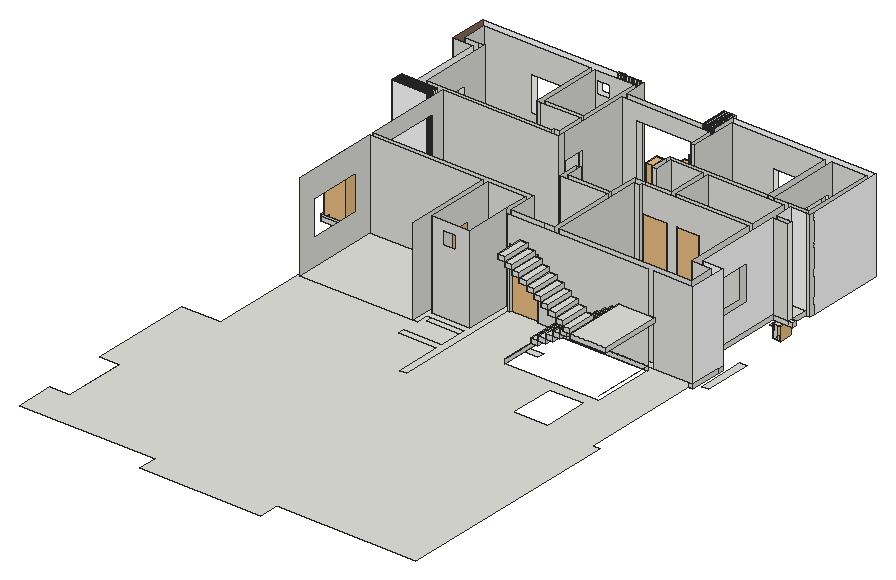
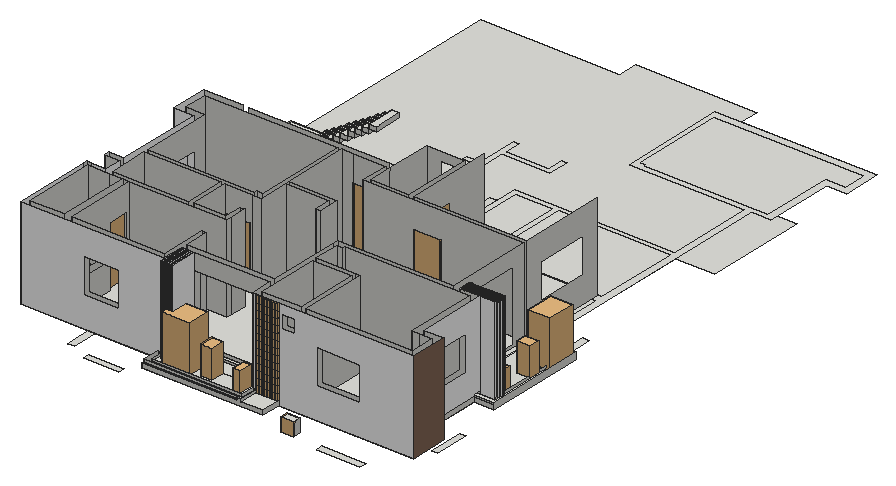
# SketchUp Ruby script. Lengths in inches.
U = 1.inch
M = Sketchup.active_model
def pt(a) = Geom::Point3d.new(a.map { |v| v * U })
def face(e, loops, mat)
  f = e.add_face(loops[0].map { |a| pt(a) })
  loops[1..].each { |l| e.add_face(l.map { |a| pt(a) }).erase! }
  f.material = f.back_material = mat if mat
  f
end
# faces: each face lists its corners as indices into pts; further lists are holes
def faces(e, pts, list, mat = nil) = list.each { |f| face(e, (f[0].is_a?(Array) ? f : [f]).map { |l| l.map { |i| pts[i] } }, mat) }
# xy, xz, yz: faces in a plane at the given z, y or x. An outline is a flat list of corners, or four numbers for a rectangle; further outlines are holes
def ring(l) = l.size == 4 ? [[l[0], l[1]], [l[2], l[1]], [l[2], l[3]], [l[0], l[3]]] : l.each_slice(2).to_a
def flat(e, list, mat, &to3) = list.each { |f| face(e, (f[0].is_a?(Array) ? f : [f]).map { |l| ring(l).map { |u, v| to3.(u, v) } }, mat) }
def xy(e, z, list, mat = nil) = flat(e, list, mat) { |x, y| [x, y, z] }
def xz(e, y, list, mat = nil) = flat(e, list, mat) { |x, z| [x, y, z] }
def yz(e, x, list, mat = nil) = flat(e, list, mat) { |y, z| [x, y, z] }
def lines(e, pts, list) = list.each { |a, b| e.add_line(pt(pts[a]), pt(pts[b])) }
# prism: a flat outline (further loops are holes) pulled along v
def prism(e, loops, v, mat = nil)
  f = face(e, loops, mat); d = Geom::Vector3d.new(v.map { |x| x * U })
  f.pushpull(f.normal.samedirection?(d) ? d.length : -d.length)
end
def box(e, o, s, mat = nil) = prism(e, [[o, [o[0] + s[0], o[1], o[2]], [o[0] + s[0], o[1] + s[1], o[2]], [o[0], o[1] + s[1], o[2]]]], [0, 0, s[2]], mat)
def at(x, y, z, deg = 0) = Geom::Transformation.translation(pt([x, y, z])) * Geom::Transformation.rotation(ORIGIN, Z_AXIS, deg.degrees)
def axes(o, x, y, z) = Geom::Transformation.new([*x, 0, *y, 0, *z, 0, *pt(o).to_a, 1])
def part(name) = M.definitions.add(name)
# library, detail: a bought-in or finely detailed component or shape, given as its bounding box
def library(name, o, s) = part(name).tap { |d| box(d.entities, o, s) }
def detail(e, o, s) = box(e.add_group.entities, o, s)
def put(e, d, t, mat = nil) = e.add_instance(d, t).tap { |i| i.material = mat if mat }
def group(e, t, mat = nil) = e.add_group.tap { |g| g.transformation = t; g.material = mat if mat }.entities
root = M.entities
M.materials.add("Manhattan Creative Coating ML 1016B 24.75cm").color = [255, 255, 255]
M.materials.add("Wintan - wpa36452 29.79cm").color = [255, 255, 255]
M.materials.add("Wood Planks C01 100cm\#1").color = [136, 107, 89]
c1 = part("Stair tread \#1")
box(c1.entities,[0,0,0],[10,39,7])
c2 = part("Stair tread")
box(c2.entities,[0,0,0],[10,39,7])
c3 = part("Group\#13")
box(c3.entities,[100,0,63],[49,84,7])
put(c3.entities,c1,at(50,45,28))
put(c3.entities,c1,at(20,45,7))
put(c3.entities,c1,at(90,45,56))
put(c3.entities,c1,at(70,45,42))
put(c3.entities,c1,at(40,45,21))
put(c3.entities,c1,at(60,45,35))
put(c3.entities,c1,at(10,45,0))
put(c3.entities,c1,at(30,45,14))
put(c3.entities,c1,at(80,45,49))
put(c3.entities,c2,at(90,0,70))
put(c3.entities,c2,at(10,0,126))
put(c3.entities,c2,at(60,0,91))
put(c3.entities,c2,at(30,0,112))
put(c3.entities,c2,at(50,0,98))
put(c3.entities,c2,at(70,0,84))
put(c3.entities,c2,at(80,0,77))
put(c3.entities,c2,at(40,0,105))
put(c3.entities,c2,at(0,0,133))
put(c3.entities,c2,at(20,0,119))
c4 = library("Door 243 053",[-21.6,-2.79,-0.07],[43.2,5.58,82.64])
c5 = library("Potted Plant 02",[-16.98,-19.78,0],[30.04,38.68,37.52])
c6 = library("Tlon Light 650 Ceiling 152 007",[-12.8,-12.8,-3.78],[25.6,25.6,3.58])
c7 = part("Square rail bar")
box(c7.entities,[0,0,-1],[51.7,1,1])
c8 = part("Group\#20")
xy(c8.entities,0,[[0,0,51.7,106.6]])
xy(c8.entities,1,[[0,0,51.7,107.6]])
xz(c8.entities,0,[[0,0,51.7,1]])
xz(c8.entities,107.6,[[0,0,51.7,1]])
yz(c8.entities,0,[[0,0,107.6,1]])
yz(c8.entities,51.7,[[0,0,107.6,1]])
put(c8.entities,c7,at(0,106.6,0))
put(c8.entities,c7,at(0,0,0))
put(c8.entities,c7,at(0,103.05,0))
put(c8.entities,c7,at(0,99.49,0))
put(c8.entities,c7,at(0,95.94,0))
put(c8.entities,c7,at(0,92.39,0))
put(c8.entities,c7,at(0,88.83,0))
put(c8.entities,c7,at(0,85.28,0))
put(c8.entities,c7,at(0,81.73,0))
put(c8.entities,c7,at(0,78.17,0))
put(c8.entities,c7,at(0,74.62,0))
put(c8.entities,c7,at(0,71.07,0))
put(c8.entities,c7,at(0,67.51,0))
put(c8.entities,c7,at(0,63.96,0))
put(c8.entities,c7,at(0,60.41,0))
put(c8.entities,c7,at(0,56.85,0))
put(c8.entities,c7,at(0,53.3,0))
put(c8.entities,c7,at(0,49.75,0))
put(c8.entities,c7,at(0,46.19,0))
put(c8.entities,c7,at(0,42.64,0))
put(c8.entities,c7,at(0,39.09,0))
put(c8.entities,c7,at(0,35.53,0))
put(c8.entities,c7,at(0,31.98,0))
put(c8.entities,c7,at(0,28.43,0))
put(c8.entities,c7,at(0,24.875,0))
put(c8.entities,c7,at(0,21.32,0))
put(c8.entities,c7,at(0,17.77,0))
put(c8.entities,c7,at(0,14.21,0))
put(c8.entities,c7,at(0,10.66,0))
put(c8.entities,c7,at(0,7.11,0))
put(c8.entities,c7,at(0,3.55,0))
put(c8.entities,c7,at(0,0,0))
c9 = library("Potted Plant 13",[-10,-7.28,0],[18.93,15.17,39.22])
c10 = library("Potted Plant 50-12",[-6.11,-5.26,0],[11.24,10.56,13.41])
c11 = part("Rectangular column")
box(c11.entities,[0,16,0],[27,1,119.8])
box(c11.entities,[0,3.56,0],[27,1,120])
box(c11.entities,[0,1.78,0],[27,1,120])
box(c11.entities,[0,14.22,0],[27,1,119.8])
box(c11.entities,[0,5.33,0],[27,1,120])
box(c11.entities,[0,7.11,0],[27,1,120])
box(c11.entities,[0,10.67,0],[27,1,120.2])
box(c11.entities,[0,12.44,0],[27,1,119.8])
box(c11.entities,[0,0,0],[27,1,120])
xy(c11.entities,0,[[0,8.89,27,9.89]])
xy(c11.entities,120,[[0,8.89,27,9.89]])
xz(c11.entities,8.89,[[0,0,27,120]])
xz(c11.entities,9.89,[[0,0,27,120]])
yz(c11.entities,0,[[8.89,0,9.89,120]],"Wintan - wpa36452 29.79cm")
yz(c11.entities,27,[[8.89,0,9.89,120]])
c12 = library("Window Crafter Awning 2",[0,-9.5,0],[17.5,11.27,18])
c13 = part("Decorative grille insert")
p = [[0.961,0,5],[0.961,0,4.995]]
lines(c13.entities,p,[[0,1]])
detail(c13.entities,[0,0,0],[4.12,1.8,10])
xy(root,336,[[1843.02,926.67,1852.02,998.67],[2008.02,962.67,2014.02,986.67],[2078.52,980.67,2117.52,989.67],[1966.02,1022.67,2002.02,1028.67],[2294.52,1040.67,2303.52,1106.67],
  [2149.02,1121.67,2181.02,1127.67],[2195.52,1121.67,2225.52,1127.67],[2005.02,1160.17,2011.02,1190.17],[1816.02,1172.67,1825.02,1220.67],[2267.52,1190.67,2276.52,1220.67],
  [1954.02,1193.67,1978.02,1199.67],[2267.52,1232.67,2276.52,1280.67],[1863.02,1286.67,1923.02,1295.67],[2195.52,1286.67,2243.52,1295.67]])
xy(root,342,[[2029.77,917.67,2047.27,926.67],[2294.52,1162.17,2303.52,1179.67],[1953.02,1286.67,1970.52,1295.67]])
xy(root,351,[[1843.02,1046.67,1852.02,1130.67],[2031.27,1256.67,2115.27,1265.67]])
xy(root,360,[[2294.52,1162.17,2303.52,1179.67],[1953.02,1286.67,1970.52,1295.67]])
xy(root,372,[[[1975.05,473.67,1975.05,500.67,1789.02,500.67,1789.02,551.67,1816.02,551.67,1816.02,637.17,1789.02,637.17,1789.02,778.17,1843.02,778.17,1843.02,1018.17,1789.02,1018.17,1789.02,1159.17,1816.02,1159.17,1816.02,1244.67,1789.02,1244.67,1789.02,1295.67,1975.05,1295.67,1975.05,1322.67,2141.52,1322.67,2141.52,1295.67,2330.52,1295.67,2330.52,1181.67,2324.52,1181.67,2324.52,1157.7,2330.52,1157.7,2330.52,1151.7,2303.52,1151.7,2303.52,1031.67,2330.52,1031.67,2330.52,980.67,2324.52,980.67,2324.52,815.67,2333.52,815.67,2333.52,500.67,2141.52,500.67,2141.52,473.67],[2138.52,896.67,2267.52,980.67],[2211.52,819.67,2259.52,883.67]],[[1789.02,500.67,2011.02,500.67,2011.02,647.67,1852.02,647.67,1852.02,767.67,2072.52,767.67,2072.52,806.67,2132.52,806.67,2132.52,715.17,2066.52,715.17,2066.52,686.67,2072.52,686.67,2072.52,709.17,2132.52,709.17,2132.52,686.67,2138.52,686.67,2138.52,743.67,2158.52,743.67,2158.52,749.67,2138.52,749.67,2138.52,806.67,2324.52,806.67,2324.52,815.67,2276.52,815.67,2276.52,980.67,2330.52,980.67,2330.52,1031.67,2303.52,1031.67,2303.52,1151.7,2324.52,1151.7,2324.52,1157.7,2303.52,1157.7,2303.52,1181.67,2330.52,1181.67,2330.52,1295.67,2132.52,1295.67,2132.52,1223.67,2138.52,1223.67,2138.52,1286.67,2324.52,1286.67,2324.52,1187.67,2132.52,1187.67,2132.52,1181.67,2183.52,1181.67,2183.52,1127.67,2132.52,1127.67,2132.52,989.67,2072.52,989.67,2072.52,1028.67,1852.02,1028.67,1852.02,1148.67,2011.02,1148.67,2011.02,1256.67,2132.52,1256.67,2132.52,1265.67,2011.02,1265.67,2011.02,1295.67,1798.02,1295.67,1798.02,1286.67,1945.02,1286.67,1945.02,1193.67,2005.02,1193.67,2005.02,1157.67,1997.02,1157.67,1997.02,1154.67,1825.02,1154.67,1825.02,1253.67,1816.02,1253.67,1816.02,1148.67,1843.02,1148.67,1843.02,647.67,1816.02,647.67,1816.02,551.67,1789.02,551.67],[1852.02,773.67,1852.02,893.67,2014.02,893.67,2014.02,891.17,2017.02,891.17,2017.02,905.17,2014.02,905.17,2014.02,902.67,1852.02,902.67,1852.02,1022.67,2008.02,1022.67,2008.02,902.67,2014.02,902.67,2014.02,1022.67,2066.52,1022.67,2066.52,773.67,2014.02,773.67,2014.02,893.67,2008.02,893.67,2008.02,773.67],[2075.52,815.67,2267.52,980.67],[1798.02,509.67,1798.02,542.67,1825.02,542.67,1825.02,641.67,1997.02,641.67,1997.02,638.67,2005.02,638.67,2005.02,509.67],[2138.52,989.67,2138.52,1118.67,2146.52,1118.67,2146.52,1121.67,2294.52,1121.67,2294.52,1022.67,2321.52,1022.67,2321.52,989.67],[2189.52,1127.67,2294.52,1181.67],[1951.02,1199.67,2005.02,1286.67]],[2014.02,917.67,2066.52,926.67],[2066.52,1081.17,2132.52,1081.17,2132.52,1087.17,2072.52,1087.17,2072.52,1109.67,2066.52,1109.67],[2132.52,1157.67,2138.52,1181.67],
  [2267.52,1187.67,2276.52,1286.67],[1789.02,1244.67,1816.02,1244.67,1816.02,1253.67,1798.02,1253.67,1798.02,1295.67,1789.02,1295.67]])
xy(root,378,[[2066.52,806.67,2075.52,806.67,2075.52,980.67,2078.52,980.67,2078.52,989.67,2072.52,989.67,2072.52,1028.67,2002.02,1028.67,2002.02,1022.67,2008.02,1022.67,2008.02,986.67,2014.02,986.67,2014.02,1022.67,2066.52,1022.67,2066.52,926.67,2014.02,926.67,2014.02,962.67,2008.02,962.67,2008.02,902.67,2014.02,902.67,2014.02,917.67,2066.52,917.67,2066.52,878.67,2014.02,878.67,2014.02,869.67,2066.52,869.67],[1852.02,902.67,2008.02,902.67,2008.02,962.67,2014.02,962.67,2014.02,986.67,2008.02,986.67,2008.02,1022.67,2002.02,1022.67,2002.02,1028.67,1966.02,1028.67,1966.02,1022.67,1852.02,1022.67],[2014.02,926.67,2066.52,1022.67],[2132.52,980.67,2330.52,980.67,2330.52,1022.67,2321.52,1022.67,2321.52,989.67,2138.52,989.67,2138.52,1118.67,2132.52,1118.67],[2072.52,989.67,2132.52,989.67,2132.52,1081.17,2066.52,1081.17,2066.52,1109.67,2072.52,1109.67,2072.52,1087.17,2132.52,1087.17,2132.52,1127.67,2149.02,1127.67,2149.02,1121.67,2146.52,1121.67,2146.52,1118.67,2138.52,1118.67,2138.52,989.67,2321.52,989.67,2321.52,1022.67,2294.52,1022.67,2294.52,1121.67,2225.52,1121.67,2225.52,1127.67,2195.52,1127.67,2195.52,1121.67,2181.02,1121.67,2181.02,1127.67,2183.52,1127.67,2183.52,1181.67,2138.52,1181.67,2138.52,1157.67,2132.52,1157.67,2132.52,1187.67,2267.52,1187.67,2267.52,1190.67,2276.52,1190.67,2276.52,1220.67,2267.52,1220.67,2267.52,1286.67,2138.52,1286.67,2138.52,1223.67,2132.52,1223.67,2132.52,1256.67,2011.02,1256.67,2011.02,1148.67,1852.02,1148.67,1852.02,1028.67,2072.52,1028.67],
  [1852.02,1022.67,1966.02,1028.67],[2294.52,1022.67,2330.52,1022.67,2330.52,1031.67,2303.52,1031.67,2303.52,1151.7,2324.52,1151.7,2324.52,1157.7,2303.52,1157.7,2303.52,1181.67,2294.52,1181.67],[1795.02,1024.17,1843.02,1148.67],[2189.52,1127.67,2294.52,1181.67],[2324.52,1151.7,2330.52,1157.7],
  [1825.02,1154.67,1997.02,1154.67,1997.02,1157.67,2005.02,1157.67,2005.02,1160.17,2011.02,1160.17,2011.02,1190.17,2005.02,1190.17,2005.02,1193.67,1978.02,1193.67,1978.02,1199.67,1954.02,1199.67,1954.02,1193.67,1945.02,1193.67,1945.02,1286.67,1798.02,1286.67,1798.02,1253.67,1825.02,1253.67],[2303.52,1157.7,2324.52,1181.67],[2276.52,1187.67,2324.52,1286.67],[1951.02,1199.67,2005.02,1286.67],[2011.02,1265.67,2132.52,1286.67],
  [2011.02,1286.67,2132.52,1286.67,2132.52,1295.67,2135.52,1295.67,2135.52,1313.67,2011.02,1313.67],[1975.05,1295.67,2005.02,1322.67],[2011.02,1319.67,2141.52,1322.67]])
xz(root,926.67,[[[2014.02,378,2066.52,498],[2029.77,468,2047.27,486]]])
xz(root,962.67,[[2008.02,378,2014.02,462]])
xz(root,980.67,[[2138.52,372,2267.52,378],[2324.52,372,2330.52,378],[2075.52,378,2078.52,378,2078.52,462,2117.52,462,2117.52,378,2267.52,378,2267.52,498,2075.52,498],[2276.52,378,2330.52,498]])
xz(root,986.67,[[2008.02,378,2014.02,462]])
xz(root,989.67,[[2072.52,378,2072.52,498,2117.52,498,2117.52,462,2078.52,462,2078.52,378],[2117.52,378,2132.52,498],[2138.52,378,2321.52,498]])
xz(root,1018.17,[[1789.02,372,1843.02,378],[1789.02,378,1843.02,381]])
xz(root,1022.67,[[1852.02,378,1966.02,378,1966.02,462,2002.02,462,2002.02,378,2008.02,378,2008.02,498,1852.02,498],[2014.02,378,2066.52,498],[2294.52,378,2321.52,498]])
xz(root,1024.17,[[1795.02,378,1843.02,381]])
xz(root,1028.67,[[1852.02,378,1852.02,498,2072.52,498,2072.52,378,2002.02,378,2002.02,462,1966.02,462,1966.02,378]])
xz(root,1031.67,[[2303.52,372,2330.52,378]])
xz(root,1031.67,[[2303.52,378,2330.52,498]],"Manhattan Creative Coating ML 1016B 24.75cm")
xz(root,1081.17,[[2066.52,378,2132.52,498]])
xz(root,1087.17,[[2072.52,378,2132.52,498]])
xz(root,1109.67,[[2066.52,378,2072.52,498]])
xz(root,1118.67,[[2138.52,378,2146.52,498]])
xz(root,1121.67,[[2146.52,378,2149.02,378,2149.02,462,2181.02,462,2181.02,378,2195.52,378,2195.52,462,2225.52,462,2225.52,378,2294.52,378,2294.52,498,2146.52,498]])
xz(root,1127.67,[[2132.52,378,2146.52,498],[2146.52,378,2146.52,498,2183.52,498,2183.52,378,2181.02,378,2181.02,462,2149.02,462,2149.02,378],[2189.52,378,2189.52,498,2294.52,498,2294.52,378,2225.52,378,2225.52,462,2195.52,462,2195.52,378]])
xz(root,1148.67,[[1795.02,378,1816.02,381],[1816.02,378,1843.02,498],[1852.02,378,2011.02,498]])
xz(root,1151.7,[[2303.52,372,2324.52,378],[2324.52,372,2330.52,378],[2303.52,378,2324.52,498]])
xz(root,1154.67,[[1825.02,378,1997.02,498]])
xz(root,1157.67,[[1997.02,378,2005.02,498],[2132.52,378,2138.52,498]])
xz(root,1157.7,[[2324.52,372,2330.52,378],[2303.52,378,2324.52,498]])
xz(root,1159.17,[[1789.02,372,1816.02,378],[1789.02,378,1816.02,381]])
xz(root,1160.17,[[2005.02,378,2011.02,462]])
xz(root,1162.17,[[2294.52,342,2303.52,360]])
xz(root,1179.67,[[2294.52,342,2303.52,360]])
xz(root,1181.67,[[2324.52,372,2330.52,498],[2138.52,378,2183.52,498],[2189.52,378,2294.52,498]])
xz(root,1181.67,[[2303.52,378,2324.52,498]],"Manhattan Creative Coating ML 1016B 24.75cm")
xz(root,1187.67,[[2132.52,378,2267.52,498],[2267.52,378,2276.52,498],[2276.52,378,2294.52,498],[2294.52,378,2324.52,498]])
xz(root,1190.17,[[2005.02,378,2011.02,462]])
xz(root,1190.67,[[2267.52,378,2276.52,462]])
xz(root,1193.67,[[1945.02,378,1951.02,498],[1951.02,378,1954.02,378,1954.02,462,1978.02,462,1978.02,378,2005.02,378,2005.02,498,1951.02,498]])
xz(root,1199.67,[[1951.02,378,1951.02,498,2005.02,498,2005.02,378,1978.02,378,1978.02,462,1954.02,462,1954.02,378]])
xz(root,1220.67,[[2267.52,378,2276.52,462]])
xz(root,1223.67,[[2132.52,378,2138.52,498]])
xz(root,1244.67,[[1789.02,372,1816.02,378],[1789.02,378,1816.02,498]])
xz(root,1253.67,[[1798.02,378,1816.02,498],[1816.02,378,1825.02,498]])
xz(root,1256.67,[[[2011.02,378,2132.52,498],[2031.27,381,2115.27,477]]])
xz(root,1265.67,[[[2011.02,378,2132.52,498],[2031.27,381,2115.27,477]]])
xz(root,1286.67,[[[1798.02,378,1945.02,498],[1863.02,414,1923.02,462]],[[1951.02,378,2005.02,498],[1953.02,468,1970.52,486]],[[2138.52,378,2267.52,498],[2195.52,414,2243.52,462]],[2276.52,378,2324.52,498]])
xz(root,1295.67,[[[1789.02,372,1789.02,498,2011.02,498,2011.02,381,2005.02,381,2005.02,378,1975.05,378,1975.05,372],[1863.02,414,1923.02,462],[1953.02,468,1970.52,486]],[[2141.52,372,2141.52,381,2135.52,381,2135.52,378,2132.52,378,2132.52,498,2330.52,498,2330.52,372],[2195.52,414,2243.52,462]]],"Manhattan Creative Coating ML 1016B 24.75cm")
xz(root,1313.67,[[2011.02,378,2135.52,381]])
xz(root,1319.67,[[2011.02,378,2141.52,381]])
xz(root,1322.67,[[1975.05,372,1975.05,378,2005.02,378,2005.02,381,2011.02,381,2011.02,378,2141.52,378,2141.52,372]])
yz(root,1789.02,[[1018.17,372,1159.17,381]])
yz(root,1789.02,[[1244.67,372,1295.67,498]],"Wood Planks C01 100cm\#1")
yz(root,1795.02,[[1024.17,378,1148.67,381]])
yz(root,1798.02,[[1253.67,378,1286.67,498]])
yz(root,1816.02,[[1159.17,372,1244.67,378]])
yz(root,1816.02,[[[1159.17,378,1159.17,381,1148.67,381,1148.67,498,1244.67,498,1244.67,378],[1172.67,414,1220.67,462]]],"Manhattan Creative Coating ML 1016B 24.75cm")
yz(root,1825.02,[[[1154.67,378,1253.67,498],[1172.67,414,1220.67,462]]])
yz(root,1852.02,[[[902.67,378,1022.67,498],[926.67,414,998.67,462]],[[1028.67,378,1148.67,498],[1046.67,381,1130.67,477]]])
yz(root,1945.02,[[1193.67,378,1286.67,498]])
yz(root,1951.02,[[1199.67,378,1286.67,498]])
yz(root,1953.02,[[1286.67,342,1295.67,360]])
yz(root,1954.02,[[1193.67,378,1199.67,462]])
yz(root,1966.02,[[1022.67,378,1028.67,462]])
yz(root,1970.52,[[1286.67,342,1295.67,360]])
yz(root,1975.05,[[1295.67,372,1322.67,378]])
yz(root,1978.02,[[1193.67,378,1199.67,462]])
yz(root,1997.02,[[1154.67,378,1157.67,498]])
yz(root,2002.02,[[1022.67,378,1028.67,462]])
yz(root,2005.02,[[1157.67,378,1157.67,498,1193.67,498,1193.67,378,1190.17,378,1190.17,462,1160.17,462,1160.17,378],[1199.67,378,1286.67,498],[1295.67,378,1322.67,381]])
yz(root,2008.02,[[902.67,378,902.67,498,1022.67,498,1022.67,378,986.67,378,986.67,462,962.67,462,962.67,378]])
yz(root,2011.02,[[1148.67,378,1157.67,498],[1157.67,378,1160.17,378,1160.17,462,1190.17,462,1190.17,378,1256.67,378,1256.67,498,1157.67,498],[1265.67,378,1295.67,498],[1295.67,378,1313.67,381],[1319.67,378,1322.67,381]])
yz(root,2014.02,[[926.67,378,962.67,378,962.67,462,986.67,462,986.67,378,1022.67,378,1022.67,498,926.67,498]])
yz(root,2066.52,[[926.67,378,989.67,498],[989.67,378,1022.67,498],[1081.17,378,1109.67,498]])
yz(root,2072.52,[[989.67,378,1028.67,498],[1087.17,378,1109.67,498]])
yz(root,2078.52,[[980.67,378,989.67,462]])
yz(root,2117.52,[[980.67,378,989.67,462]])
yz(root,2132.52,[[989.67,378,1081.17,498],[1081.17,378,1087.17,498],[1087.17,378,1127.67,498],[1157.67,378,1181.67,498],[1181.67,378,1187.67,498],
  [1223.67,378,1256.67,498],[1265.67,378,1295.67,498]])
yz(root,2135.52,[[1295.67,378,1313.67,381]])
yz(root,2138.52,[[896.67,372,980.67,378],[989.67,378,1118.67,498],[1157.67,378,1181.67,498],[1223.67,378,1286.67,498]])
yz(root,2141.52,[[1295.67,372,1322.67,372,1322.67,378,1319.67,378,1319.67,381,1295.67,381]])
yz(root,2146.52,[[1118.67,378,1121.67,498]])
yz(root,2149.02,[[1121.67,378,1127.67,462]])
yz(root,2181.02,[[1121.67,378,1127.67,462]])
yz(root,2183.52,[[1127.67,378,1181.67,498]])
yz(root,2189.52,[[1127.67,378,1181.67,498]])
yz(root,2195.52,[[1121.67,378,1127.67,462]])
yz(root,2225.52,[[1121.67,378,1127.67,462]])
yz(root,2267.52,[[[1187.67,378,1187.67,498,1286.67,498,1286.67,378,1220.67,378,1220.67,462,1190.67,462,1190.67,378],[1232.67,414,1280.67,462]]])
yz(root,2276.52,[[[1187.67,378,1190.67,378,1190.67,462,1220.67,462,1220.67,378,1286.67,378,1286.67,498,1187.67,498],[1232.67,414,1280.67,462]]])
yz(root,2294.52,[[[1022.67,378,1121.67,498],[1040.67,414,1106.67,462]],[[1127.67,378,1181.67,498],[1162.17,468,1179.67,486]]])
yz(root,2303.52,[[1031.67,372,1151.7,378]])
yz(root,2303.52,[[[1031.67,378,1151.7,498],[1040.67,414,1106.67,462]],[[1157.7,378,1181.67,498],[1162.17,468,1179.67,486]]],"Manhattan Creative Coating ML 1016B 24.75cm")
yz(root,2321.52,[[989.67,378,1022.67,498]])
yz(root,2324.52,[[1157.7,372,1181.67,378],[1187.67,378,1286.67,498]])
yz(root,2324.52,[[1151.7,378,1157.7,498]],"Manhattan Creative Coating ML 1016B 24.75cm")
yz(root,2330.52,[[980.67,372,1022.67,378],[1022.67,372,1031.67,378],[1151.7,372,1157.7,378],[1181.67,372,1187.67,498]])
yz(root,2330.52,[[1187.67,372,1295.67,498],[980.67,378,1031.67,498]],"Manhattan Creative Coating ML 1016B 24.75cm")
p = [[2138.52,896.67,378],[2138.52,980.67,378],[2267.52,980.67,378],[2267.52,896.67,378]]
lines(root,p,[[0,1],[1,2],[2,3]])
put(root,c3,axes([2128.52,896.67,378],[1,0,0],[0,1,0],[0,0,0.9]))
put(root,c4,axes([2011.02,974.68,378.07],[0,-0.55585,0],[1.07698,0,0],[0,0,1.01843]))
put(root,c4,axes([2097.77,985.74,378.07],[0.9143,0,0],[0,0.74,0],[0,0,1.01843]))
put(root,c4,axes([1984.02,1027.84,377.91],[0.83329,0,0],[0,0.74,0],[0,0,1.01843]))
put(root,c5,axes([1806.01,1043.12,378],[1,0,0],[0,1,0],[0,0,1.71]))
put(root,c6,axes([1817.33,1048.52,370.24],[0.44,0,0],[0,0.44,0],[0,0,0.44]))
put(root,c8,at(1791.32,1022.61,371))
put(root,c9,at(1804.9375,1080.65,378))
put(root,c6,axes([1817.33,1094.72,370.24],[0.44,0,0],[0,0.44,0],[0,0,0.44]))
put(root,c4,axes([2210.52,1123.74,378.07],[0.69441,0,0],[0,0.74,0],[0,0,1.01843]))
put(root,c4,axes([2165.02,1123.74,378.07],[0.7407,0,0],[0,0.74,0],[0,0,1.01843]))
put(root,c10,axes([1808.5,1124.17,378],[1.65,0,0],[0,1,0],[0,0,2]))
put(root,c11,axes([1795.02,1131.67,378],[1.77778,0,0],[0,1,0],[0,0,1]),"Wintan - wpa36452 29.79cm")
put(root,c12,at(2296.3,1162.17,342,90))
put(root,c4,axes([1966.02,1196.98,377.91],[0.55552,0,0],[0,0.74,0],[0,0,1.01843]))
put(root,c4,axes([2273.94,1205.63,377.86],[0,-0.69441,0],[0.74,0,0],[0,0,1.01843]))
put(root,c6,axes([2077.86,1282.86,369.8125],[0.44,0,0],[0,0.44,0],[0,0,0.44]))
put(root,c6,axes([2034,1282.86,369.8125],[0.44,0,0],[0,0.44,0],[0,0,0.44]))
put(root,c11,axes([2132.52,1265.67,378],[0,1.33704,0],[-1,0,0],[0,0,0.99769]),"Wintan - wpa36452 29.79cm")
put(root,c8,axes([2011.02,1301.77,370.6],[0,-0.69826,0],[0.97119,0,0],[0,0,1]))
put(root,c12,at(1970.52,1288.45,342,180))
put(root,c5,axes([2104.14,1297.51,378],[0,1,0],[-1,0,0],[0,0,1.71]))
put(root,c9,at(2066.61,1296.4375,378,90))
g1 = group(root,at(1975.05,1295.67,378))
put(g1,c13,axes([0,0,0],[0.90915,0,0],[0,1,0],[0,0,0.92482]))
put(g1,c13,axes([3.75,0,0],[0.90915,0,0],[0,1,0],[0,0,0.92482]))
put(g1,c13,axes([7.49,0,0],[0.90915,0,0],[0,1,0],[0,0,0.92482]))
put(g1,c13,axes([11.24,0,0],[0.90915,0,0],[0,1,0],[0,0,0.92482]))
put(g1,c13,axes([14.99,0,0],[0.90915,0,0],[0,1,0],[0,0,0.92482]))
put(g1,c13,axes([18.73,0,0],[0.90915,0,0],[0,1,0],[0,0,0.92482]))
put(g1,c13,axes([22.48,0,0],[0.90915,0,0],[0,1,0],[0,0,0.92482]))
put(g1,c13,axes([26.23,0,0],[0.90915,0,0],[0,1,0],[0,0,0.92482]))
put(g1,c13,axes([0,0,9.25],[0.90915,0,0],[0,1,0],[0,0,0.92482]))
put(g1,c13,axes([26.23,0,9.25],[0.90915,0,0],[0,1,0],[0,0,0.92482]))
put(g1,c13,axes([22.48,0,9.25],[0.90915,0,0],[0,1,0],[0,0,0.92482]))
put(g1,c13,axes([18.73,0,9.25],[0.90915,0,0],[0,1,0],[0,0,0.92482]))
put(g1,c13,axes([11.24,0,9.25],[0.90915,0,0],[0,1,0],[0,0,0.92482]))
put(g1,c13,axes([14.99,0,9.25],[0.90915,0,0],[0,1,0],[0,0,0.92482]))
put(g1,c13,axes([3.75,0,9.25],[0.90915,0,0],[0,1,0],[0,0,0.92482]))
put(g1,c13,axes([7.49,0,9.25],[0.90915,0,0],[0,1,0],[0,0,0.92482]))
put(g1,c13,axes([0,0,18.5],[0.90915,0,0],[0,1,0],[0,0,0.92482]))
put(g1,c13,axes([26.23,0,18.5],[0.90915,0,0],[0,1,0],[0,0,0.92482]))
put(g1,c13,axes([22.48,0,18.5],[0.90915,0,0],[0,1,0],[0,0,0.92482]))
put(g1,c13,axes([18.73,0,18.5],[0.90915,0,0],[0,1,0],[0,0,0.92482]))
put(g1,c13,axes([11.24,0,18.5],[0.90915,0,0],[0,1,0],[0,0,0.92482]))
put(g1,c13,axes([14.99,0,18.5],[0.90915,0,0],[0,1,0],[0,0,0.92482]))
put(g1,c13,axes([3.75,0,18.5],[0.90915,0,0],[0,1,0],[0,0,0.92482]))
put(g1,c13,axes([7.49,0,18.5],[0.90915,0,0],[0,1,0],[0,0,0.92482]))
put(g1,c13,axes([0,0,27.74],[0.90915,0,0],[0,1,0],[0,0,0.92482]))
put(g1,c13,axes([26.23,0,27.74],[0.90915,0,0],[0,1,0],[0,0,0.92482]))
put(g1,c13,axes([22.48,0,27.74],[0.90915,0,0],[0,1,0],[0,0,0.92482]))
put(g1,c13,axes([18.73,0,27.74],[0.90915,0,0],[0,1,0],[0,0,0.92482]))
put(g1,c13,axes([11.24,0,27.74],[0.90915,0,0],[0,1,0],[0,0,0.92482]))
put(g1,c13,axes([14.99,0,27.74],[0.90915,0,0],[0,1,0],[0,0,0.92482]))
put(g1,c13,axes([3.75,0,27.74],[0.90915,0,0],[0,1,0],[0,0,0.92482]))
put(g1,c13,axes([7.49,0,27.74],[0.90915,0,0],[0,1,0],[0,0,0.92482]))
put(g1,c13,axes([0,0,36.99],[0.90915,0,0],[0,1,0],[0,0,0.92482]))
put(g1,c13,axes([26.23,0,36.99],[0.90915,0,0],[0,1,0],[0,0,0.92482]))
put(g1,c13,axes([22.48,0,36.99],[0.90915,0,0],[0,1,0],[0,0,0.92482]))
put(g1,c13,axes([18.73,0,36.99],[0.90915,0,0],[0,1,0],[0,0,0.92482]))
put(g1,c13,axes([11.24,0,36.99],[0.90915,0,0],[0,1,0],[0,0,0.92482]))
put(g1,c13,axes([14.99,0,36.99],[0.90915,0,0],[0,1,0],[0,0,0.92482]))
put(g1,c13,axes([3.75,0,36.99],[0.90915,0,0],[0,1,0],[0,0,0.92482]))
put(g1,c13,axes([7.49,0,36.99],[0.90915,0,0],[0,1,0],[0,0,0.92482]))
put(g1,c13,axes([0,0,46.24],[0.90915,0,0],[0,1,0],[0,0,0.92482]))
put(g1,c13,axes([26.23,0,46.24],[0.90915,0,0],[0,1,0],[0,0,0.92482]))
put(g1,c13,axes([22.48,0,46.24],[0.90915,0,0],[0,1,0],[0,0,0.92482]))
put(g1,c13,axes([18.73,0,46.24],[0.90915,0,0],[0,1,0],[0,0,0.92482]))
put(g1,c13,axes([11.24,0,46.24],[0.90915,0,0],[0,1,0],[0,0,0.92482]))
put(g1,c13,axes([14.99,0,46.24],[0.90915,0,0],[0,1,0],[0,0,0.92482]))
put(g1,c13,axes([3.75,0,46.24],[0.90915,0,0],[0,1,0],[0,0,0.92482]))
put(g1,c13,axes([7.49,0,46.24],[0.90915,0,0],[0,1,0],[0,0,0.92482]))
put(g1,c13,axes([0,0,55.49],[0.90915,0,0],[0,1,0],[0,0,0.92482]))
put(g1,c13,axes([26.23,0,55.49],[0.90915,0,0],[0,1,0],[0,0,0.92482]))
put(g1,c13,axes([22.48,0,55.49],[0.90915,0,0],[0,1,0],[0,0,0.92482]))
put(g1,c13,axes([18.73,0,55.49],[0.90915,0,0],[0,1,0],[0,0,0.92482]))
put(g1,c13,axes([11.24,0,55.49],[0.90915,0,0],[0,1,0],[0,0,0.92482]))
put(g1,c13,axes([14.99,0,55.49],[0.90915,0,0],[0,1,0],[0,0,0.92482]))
put(g1,c13,axes([3.75,0,55.49],[0.90915,0,0],[0,1,0],[0,0,0.92482]))
put(g1,c13,axes([7.49,0,55.49],[0.90915,0,0],[0,1,0],[0,0,0.92482]))
put(g1,c13,axes([0,0,64.74],[0.90915,0,0],[0,1,0],[0,0,0.92482]))
put(g1,c13,axes([26.23,0,64.74],[0.90915,0,0],[0,1,0],[0,0,0.92482]))
put(g1,c13,axes([22.48,0,64.74],[0.90915,0,0],[0,1,0],[0,0,0.92482]))
put(g1,c13,axes([18.73,0,64.74],[0.90915,0,0],[0,1,0],[0,0,0.92482]))
put(g1,c13,axes([11.24,0,64.74],[0.90915,0,0],[0,1,0],[0,0,0.92482]))
put(g1,c13,axes([14.99,0,64.74],[0.90915,0,0],[0,1,0],[0,0,0.92482]))
put(g1,c13,axes([3.75,0,64.74],[0.90915,0,0],[0,1,0],[0,0,0.92482]))
put(g1,c13,axes([7.49,0,64.74],[0.90915,0,0],[0,1,0],[0,0,0.92482]))
put(g1,c13,axes([0,0,73.99],[0.90915,0,0],[0,1,0],[0,0,0.92482]))
put(g1,c13,axes([26.23,0,73.99],[0.90915,0,0],[0,1,0],[0,0,0.92482]))
put(g1,c13,axes([22.48,0,73.99],[0.90915,0,0],[0,1,0],[0,0,0.92482]))
put(g1,c13,axes([18.73,0,73.99],[0.90915,0,0],[0,1,0],[0,0,0.92482]))
put(g1,c13,axes([11.24,0,73.99],[0.90915,0,0],[0,1,0],[0,0,0.92482]))
put(g1,c13,axes([14.99,0,73.99],[0.90915,0,0],[0,1,0],[0,0,0.92482]))
put(g1,c13,axes([3.75,0,73.99],[0.90915,0,0],[0,1,0],[0,0,0.92482]))
put(g1,c13,axes([7.49,0,73.99],[0.90915,0,0],[0,1,0],[0,0,0.92482]))
put(g1,c13,axes([0,0,83.23],[0.90915,0,0],[0,1,0],[0,0,0.92482]))
put(g1,c13,axes([26.23,0,83.23],[0.90915,0,0],[0,1,0],[0,0,0.92482]))
put(g1,c13,axes([22.48,0,83.23],[0.90915,0,0],[0,1,0],[0,0,0.92482]))
put(g1,c13,axes([18.73,0,83.23],[0.90915,0,0],[0,1,0],[0,0,0.92482]))
put(g1,c13,axes([11.24,0,83.23],[0.90915,0,0],[0,1,0],[0,0,0.92482]))
put(g1,c13,axes([14.99,0,83.23],[0.90915,0,0],[0,1,0],[0,0,0.92482]))
put(g1,c13,axes([3.75,0,83.23],[0.90915,0,0],[0,1,0],[0,0,0.92482]))
put(g1,c13,axes([7.49,0,83.23],[0.90915,0,0],[0,1,0],[0,0,0.92482]))
put(g1,c13,axes([0,0,92.48],[0.90915,0,0],[0,1,0],[0,0,0.92482]))
put(g1,c13,axes([26.23,0,92.48],[0.90915,0,0],[0,1,0],[0,0,0.92482]))
put(g1,c13,axes([22.48,0,92.48],[0.90915,0,0],[0,1,0],[0,0,0.92482]))
put(g1,c13,axes([18.73,0,92.48],[0.90915,0,0],[0,1,0],[0,0,0.92482]))
put(g1,c13,axes([11.24,0,92.48],[0.90915,0,0],[0,1,0],[0,0,0.92482]))
put(g1,c13,axes([14.99,0,92.48],[0.90915,0,0],[0,1,0],[0,0,0.92482]))
put(g1,c13,axes([3.75,0,92.48],[0.90915,0,0],[0,1,0],[0,0,0.92482]))
put(g1,c13,axes([7.49,0,92.48],[0.90915,0,0],[0,1,0],[0,0,0.92482]))
put(g1,c13,axes([0,0,101.73],[0.90915,0,0],[0,1,0],[0,0,0.92482]))
put(g1,c13,axes([26.23,0,101.73],[0.90915,0,0],[0,1,0],[0,0,0.92482]))
put(g1,c13,axes([22.48,0,101.73],[0.90915,0,0],[0,1,0],[0,0,0.92482]))
put(g1,c13,axes([18.73,0,101.73],[0.90915,0,0],[0,1,0],[0,0,0.92482]))
put(g1,c13,axes([11.24,0,101.73],[0.90915,0,0],[0,1,0],[0,0,0.92482]))
put(g1,c13,axes([14.99,0,101.73],[0.90915,0,0],[0,1,0],[0,0,0.92482]))
put(g1,c13,axes([3.75,0,101.73],[0.90915,0,0],[0,1,0],[0,0,0.92482]))
put(g1,c13,axes([7.49,0,101.73],[0.90915,0,0],[0,1,0],[0,0,0.92482]))
put(g1,c13,axes([0,0,110.98],[0.90915,0,0],[0,1,0],[0,0,0.92482]))
put(g1,c13,axes([26.23,0,110.98],[0.90915,0,0],[0,1,0],[0,0,0.92482]))
put(g1,c13,axes([22.48,0,110.98],[0.90915,0,0],[0,1,0],[0,0,0.92482]))
put(g1,c13,axes([18.73,0,110.98],[0.90915,0,0],[0,1,0],[0,0,0.92482]))
put(g1,c13,axes([11.24,0,110.98],[0.90915,0,0],[0,1,0],[0,0,0.92482]))
put(g1,c13,axes([14.99,0,110.98],[0.90915,0,0],[0,1,0],[0,0,0.92482]))
put(g1,c13,axes([3.75,0,110.98],[0.90915,0,0],[0,1,0],[0,0,0.92482]))
put(g1,c13,axes([7.49,0,110.98],[0.90915,0,0],[0,1,0],[0,0,0.92482]))
put(root,c10,axes([2023.09,1300,378],[0,1.65,0],[-1,0,0],[0,0,2]))
